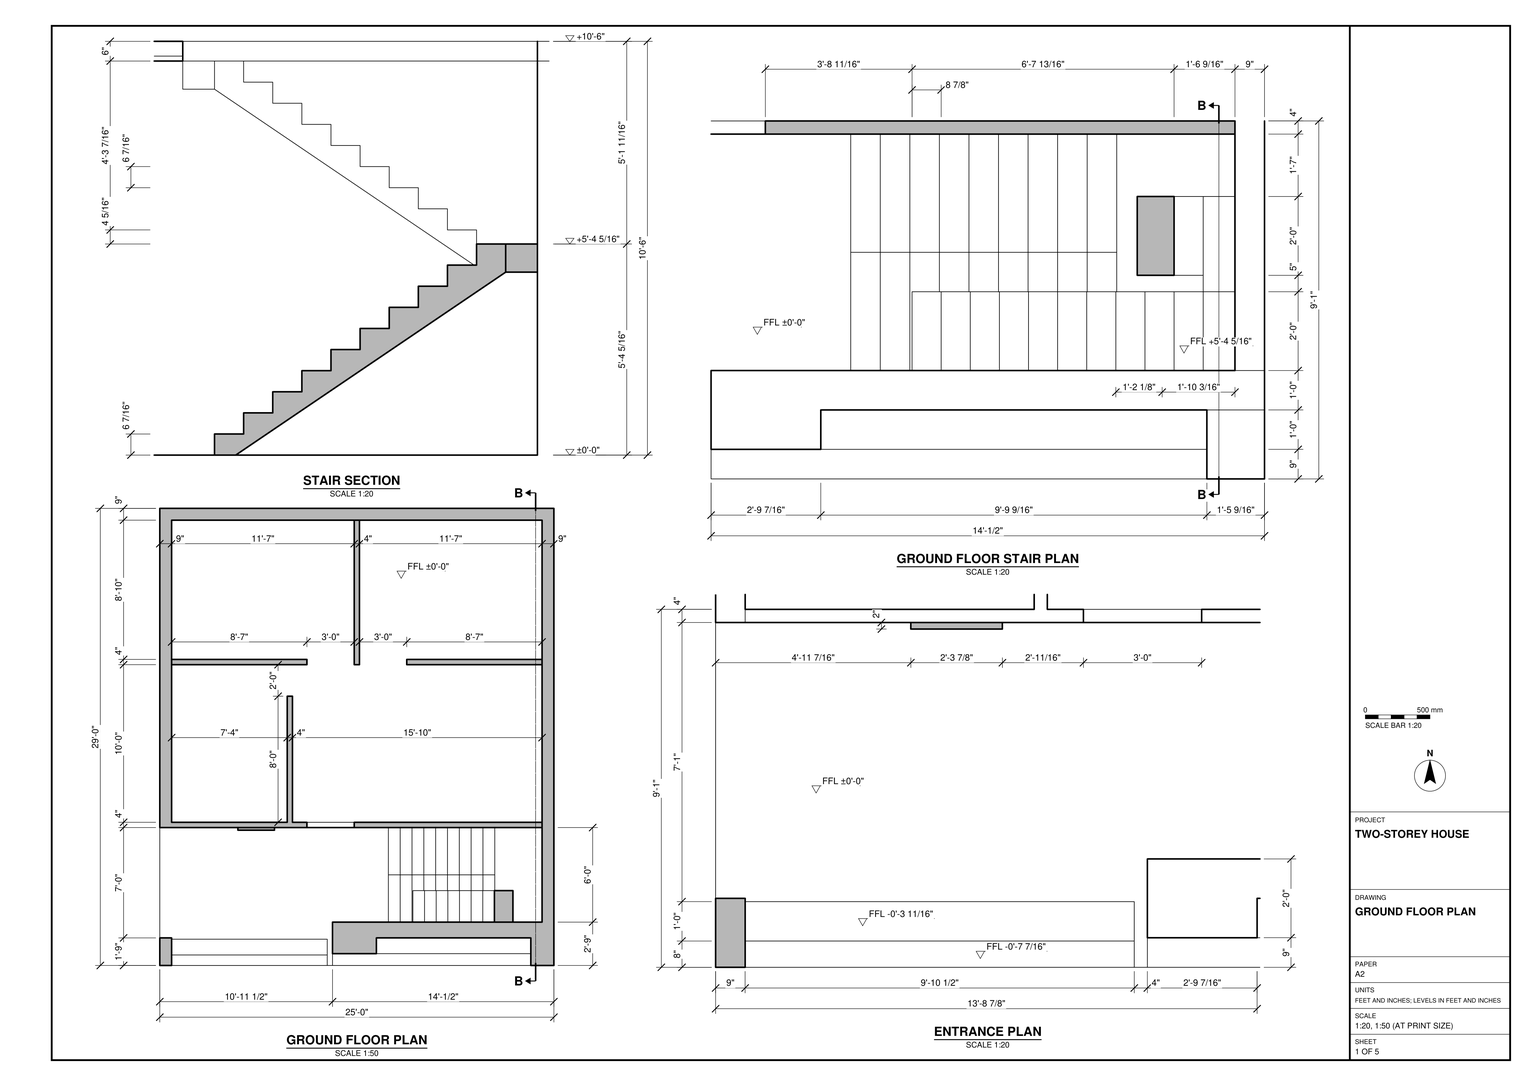
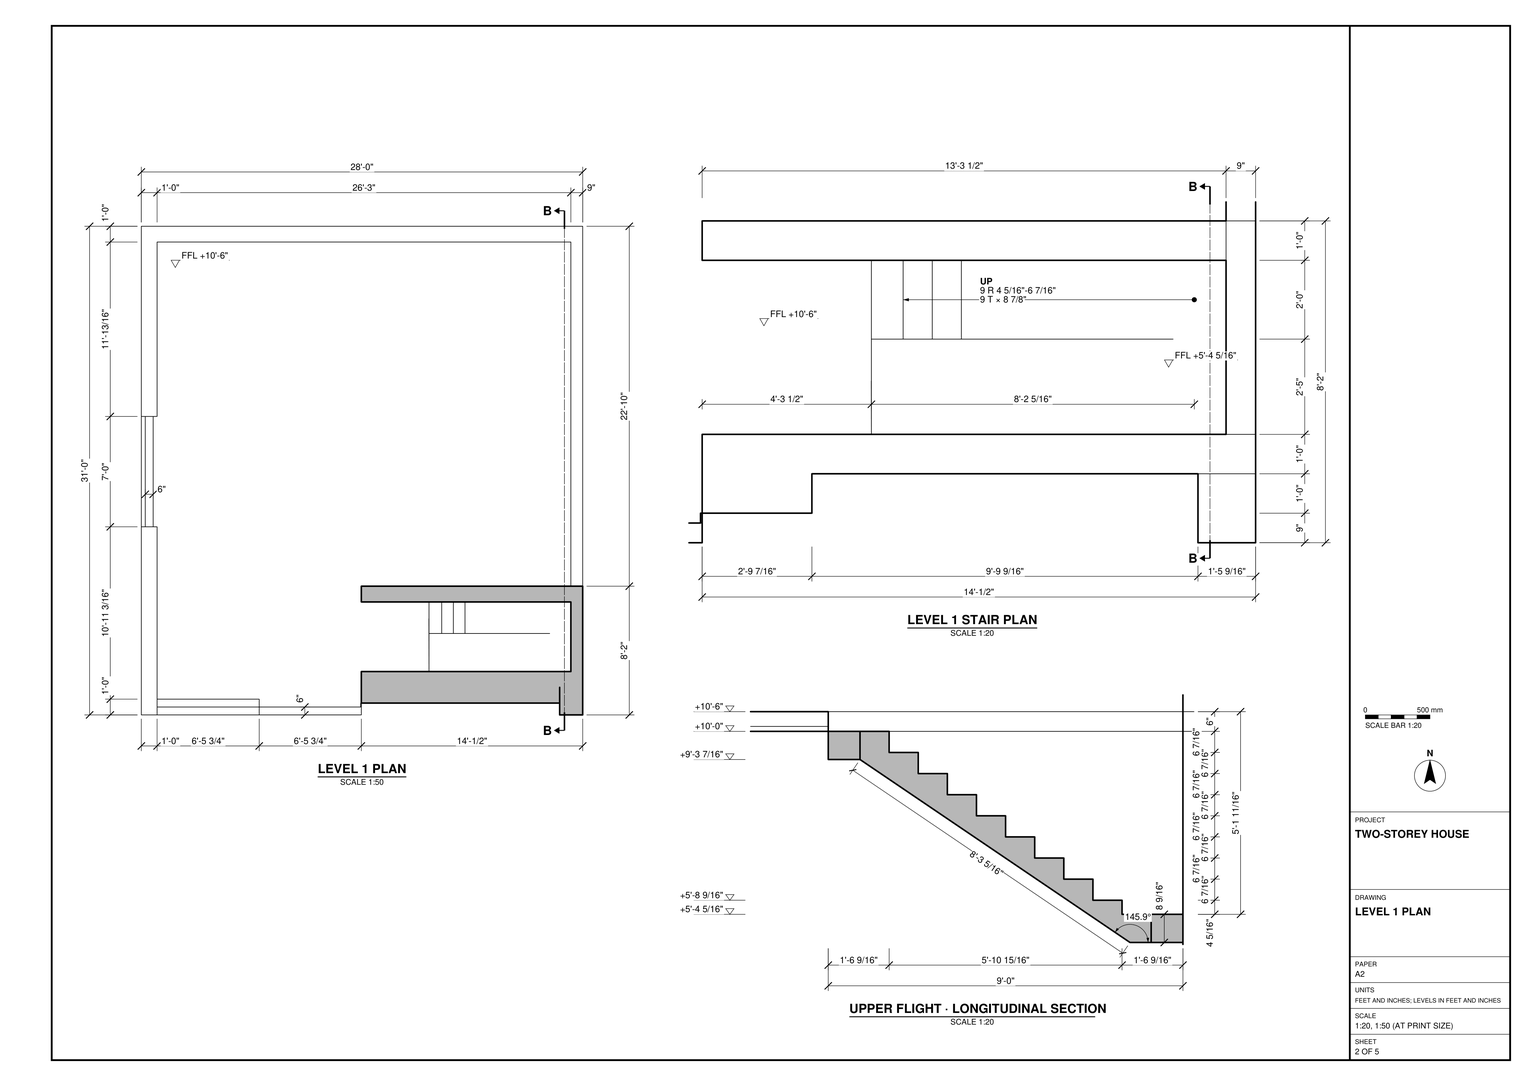
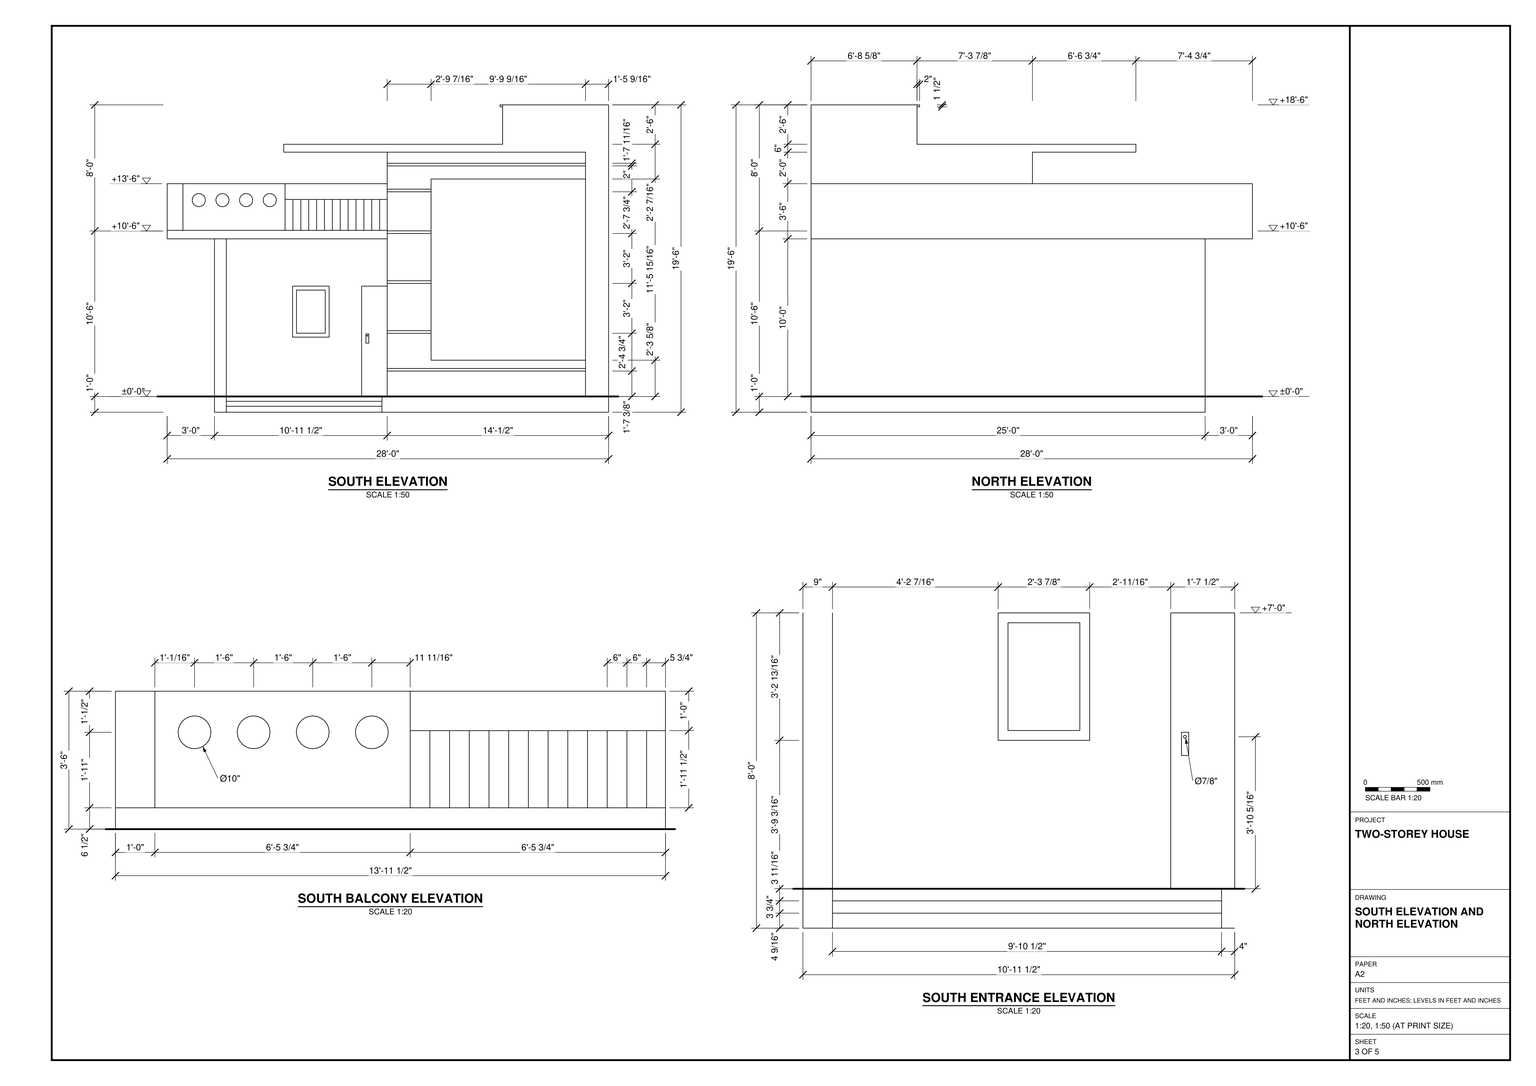
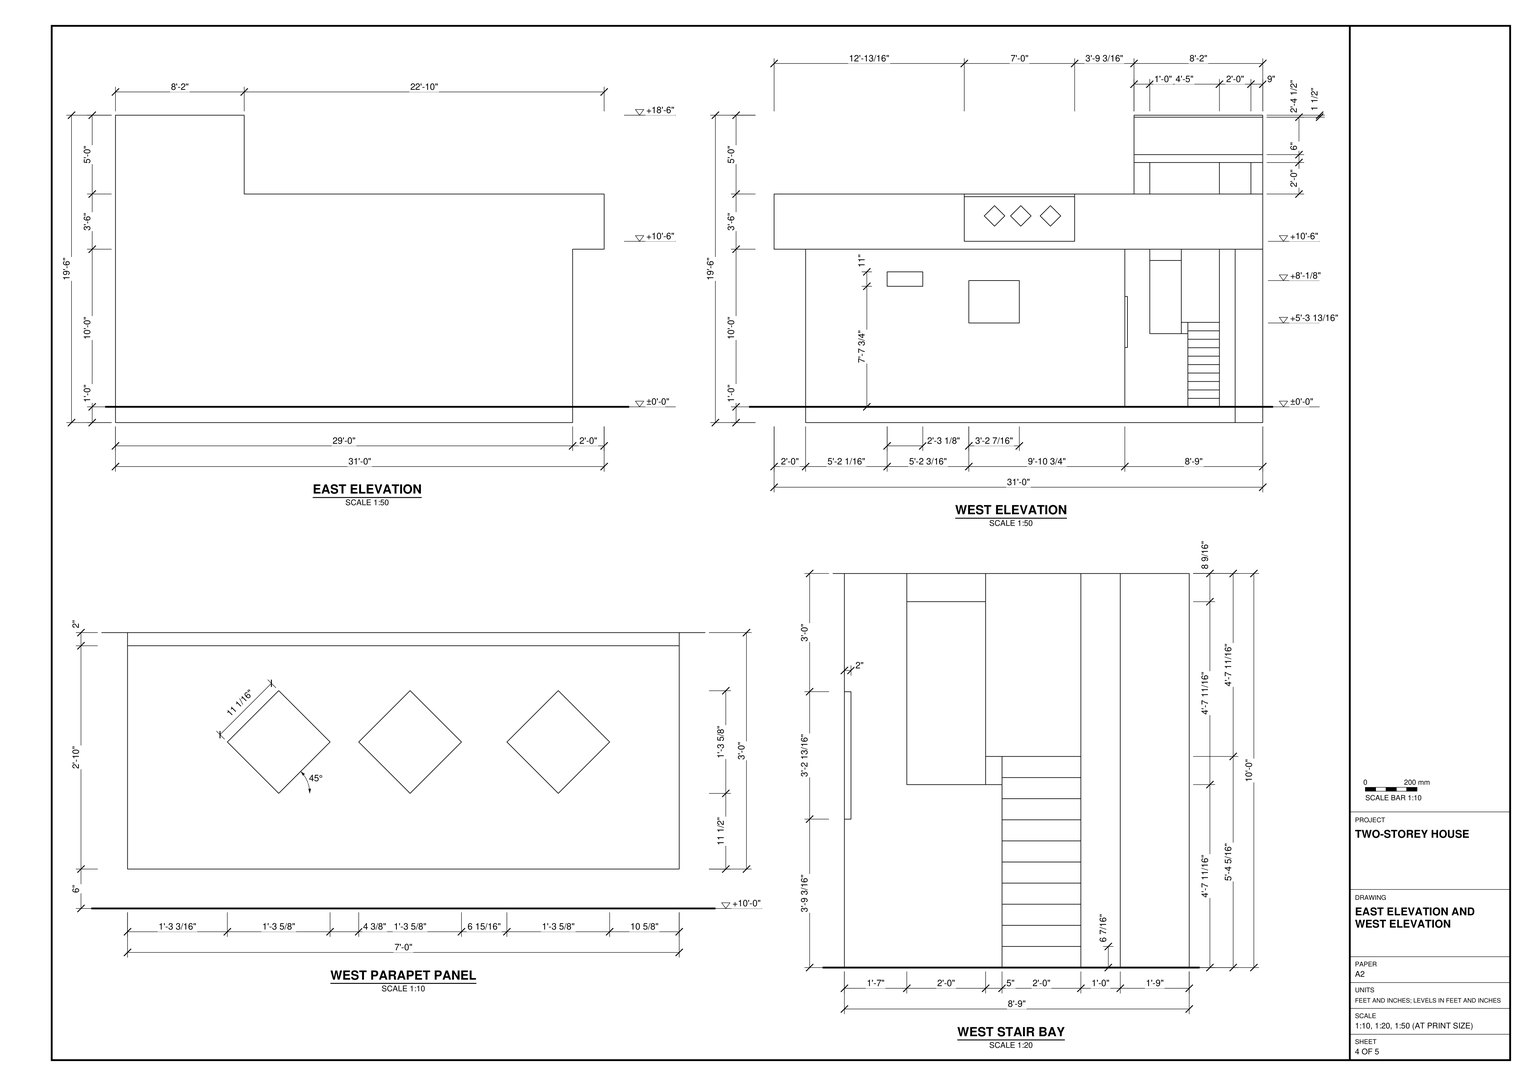
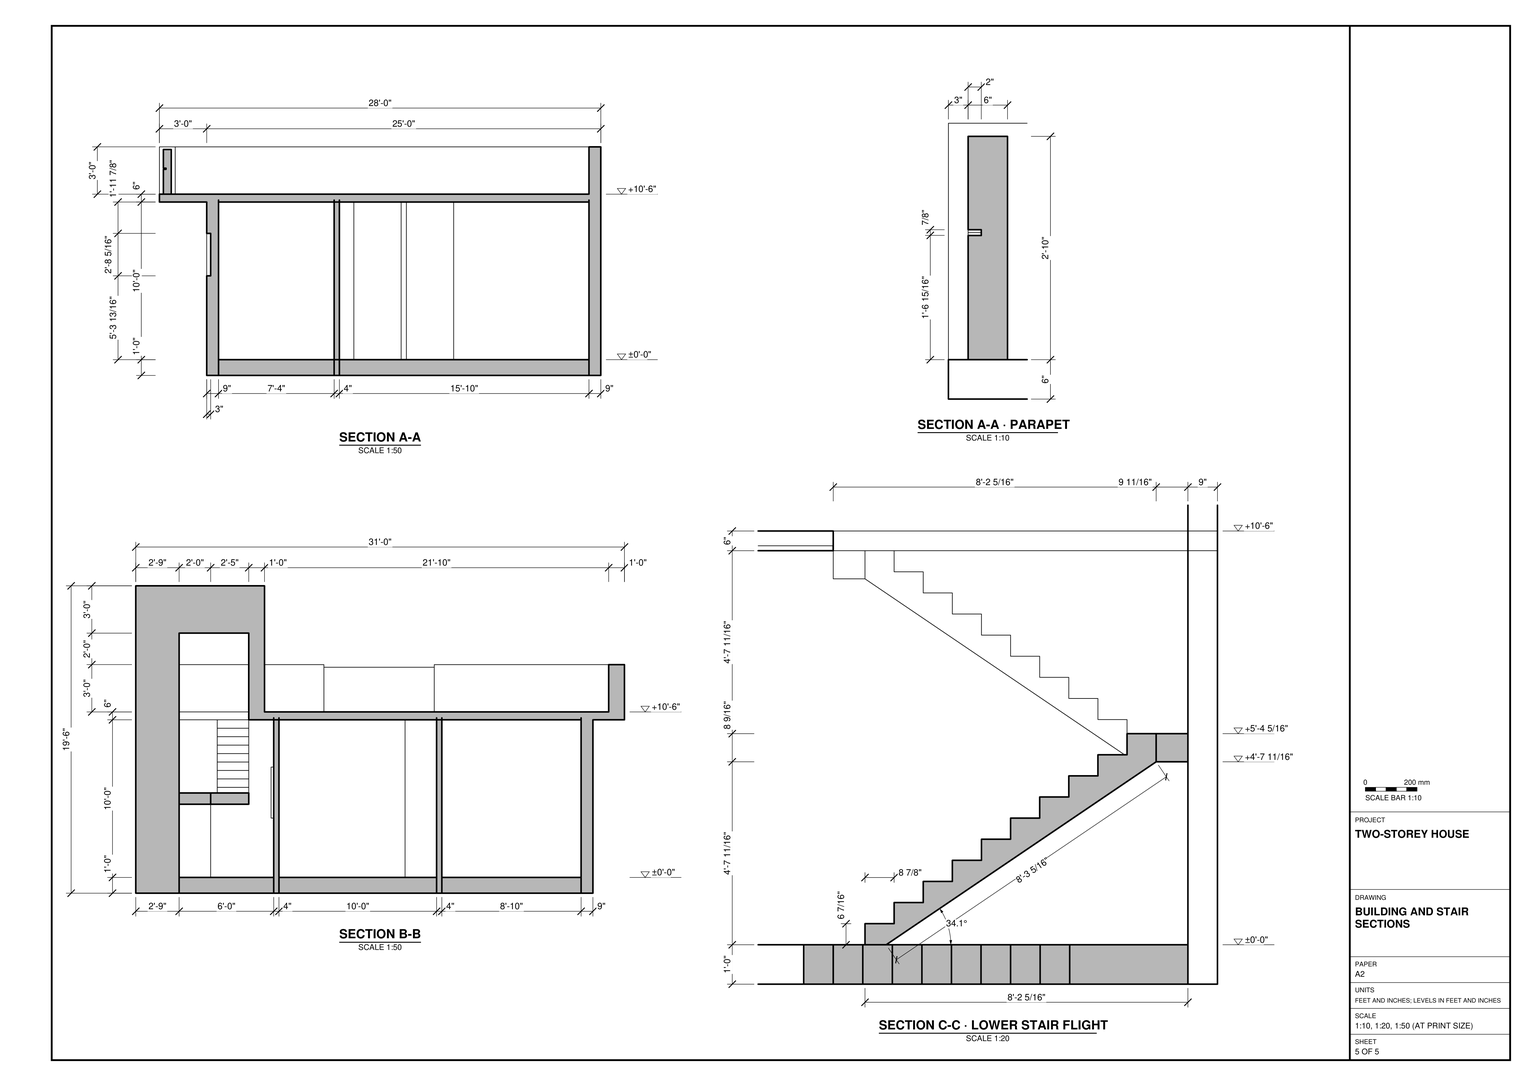
Build the house in SketchUp from task_files/diagram_01.pdf. Work in feet and inches. The complete model extents are 63'-3 1/16" along X, 31'-11 3/16" along Y and 19'-6" vertically. Use the plan dimensions for the house itself: the ground-floor footprint, including the entrance and stair area, is 25'-0" by 29'-0". Set the ground floor at ±0'-0" and the upper level at +10'-6".

Model the base, floor slabs, 9" exterior walls and 4" interior partitions. Follow the ground-floor plan for the paired rear rooms, the shorter partition in front of them and the gaps that give access between spaces. Recess the south entrance behind the balcony, with steps up to the door and a framed window to its left. Beside the entrance, build the two stair flights running in opposite directions, joined at the +5'-4 5/16" landing. Match the stepped treads and inclined undersides in section, and leave the opening for arrival at the roof terrace.

Follow the elevations for the projecting upper slab, terrace edges and taller stepped surround beside the stair. On the south balcony, distinguish the panel with circular details from the adjoining vertical railing. Keep walls, slabs, roof elements and stairs in separate groups or components; keep each furniture or joinery piece shown separate and use components for repeated parts. Any decor or loose items shown may be suitable library components. Save one SketchUp model as output_files/two_storey_house_with_its_return_stair_and_roof_terrace.skp.

# SketchUp Ruby script. Lengths in inches.
U = 1.inch
M = Sketchup.active_model
def pt(a) = Geom::Point3d.new(a.map { |v| v * U })
def face(e, loops, mat)
  f = e.add_face(loops[0].map { |a| pt(a) })
  loops[1..].each { |l| e.add_face(l.map { |a| pt(a) }).erase! }
  f.material = f.back_material = mat if mat
  f
end
# faces: each face lists its corners as indices into pts; further lists are holes
def faces(e, pts, list, mat = nil) = list.each { |f| face(e, (f[0].is_a?(Array) ? f : [f]).map { |l| l.map { |i| pts[i] } }, mat) }
# xy, xz, yz: faces in a plane at the given z, y or x. An outline is a flat list of corners, or four numbers for a rectangle; further outlines are holes
def ring(l) = l.size == 4 ? [[l[0], l[1]], [l[2], l[1]], [l[2], l[3]], [l[0], l[3]]] : l.each_slice(2).to_a
def flat(e, list, mat, &to3) = list.each { |f| face(e, (f[0].is_a?(Array) ? f : [f]).map { |l| ring(l).map { |u, v| to3.(u, v) } }, mat) }
def xy(e, z, list, mat = nil) = flat(e, list, mat) { |x, y| [x, y, z] }
def xz(e, y, list, mat = nil) = flat(e, list, mat) { |x, z| [x, y, z] }
def yz(e, x, list, mat = nil) = flat(e, list, mat) { |y, z| [x, y, z] }
def lines(e, pts, list) = list.each { |a, b| e.add_line(pt(pts[a]), pt(pts[b])) }
# prism: a flat outline (further loops are holes) pulled along v
def prism(e, loops, v, mat = nil)
  f = face(e, loops, mat); d = Geom::Vector3d.new(v.map { |x| x * U })
  f.pushpull(f.normal.samedirection?(d) ? d.length : -d.length)
end
def box(e, o, s, mat = nil) = prism(e, [[o, [o[0] + s[0], o[1], o[2]], [o[0] + s[0], o[1] + s[1], o[2]], [o[0], o[1] + s[1], o[2]]]], [0, 0, s[2]], mat)
def at(x, y, z, deg = 0) = Geom::Transformation.translation(pt([x, y, z])) * Geom::Transformation.rotation(ORIGIN, Z_AXIS, deg.degrees)
def axes(o, x, y, z) = Geom::Transformation.new([*x, 0, *y, 0, *z, 0, *pt(o).to_a, 1])
def part(name) = M.definitions.add(name)
# library, detail: a bought-in or finely detailed component or shape, given as its bounding box
def library(name, o, s) = part(name).tap { |d| box(d.entities, o, s) }
def detail(e, o, s) = box(e.add_group.entities, o, s)
def put(e, d, t, mat = nil) = e.add_instance(d, t).tap { |i| i.material = mat if mat }
def group(e, t, mat = nil) = e.add_group.tap { |g| g.transformation = t; g.material = mat if mat }.entities
root = M.entities
M.materials.add("[0006_Pink]").color = [255, 192, 203]
M.materials.add("[0017_IndianRed]").color = [205, 92, 92]
M.materials.add("[0022_Maroon]").color = [58, 0, 0]
M.materials.add("[0078_DarkSlateGray]").color = [47, 79, 79]
M.materials.add("[0081_CadetBlue]").color = [43, 73, 73]
M.materials.add("[0081_CadetBlue]1").color = [78, 130, 132]
M.materials.add("[0081_CadetBlue]2").color = [69, 115, 117]
M.materials.add("[0093_AliceBlue]").color = [240, 248, 255]
M.materials.add("[0099_LightSteelBlue]").color = [176, 196, 222]
M.materials.add("[0117_GhostWhite]").color = [248, 248, 255]
M.materials.add("[0118_Thistle]").color = [198, 175, 198]
M.materials.add("[0119_RosyBrown]").color = [247, 188, 188]
M.materials.add("[Grass Dark Green]").color = [106, 157, 55]
M.materials.add("[Stone Marble]").color = [143, 138, 136]
M.materials.add("[Stone Vein Gray]").color = [166, 165, 165]
M.materials.add("[Translucent Resin Crush Gray]").color = [184, 184, 184]
M.materials["[Translucent Resin Crush Gray]"].alpha = 0.8
M.materials.add("[Wood Veneer 01]").color = [84, 49, 25]
M.materials.add("[Wood Veneer 01]1").color = [120, 70, 37]
xy(root,-12,[[36,0,45,21],[45,0,163.47,9],[163.47,0,167.47,33],[167.47,0,336,33],[45,9,163.47,21],
  [36,21,163.47,33],[327,33,327,339,45,339,45,105,36,105,36,348,336,348,336,33],[36,33,36,105,148,105,148,109,137,109,137,205,133,205,133,109,45,109,45,229,148,229,148,233,45,233,45,339,184,339,184,229,188,229,188,339,327,339,327,233,224,233,224,229,327,229,327,109,184,109,184,105,210,105,210,33],[210,33,219,69],[219,33,228,69],
  [228,33,237,69],[237,33,246,69],[246,33,255,69],[255,33,264,69],[264,33,273,69],
  [273,33,282,69],[282,33,291,69],[291,33,327,105],[210,69,219,105],[219,69,228,105],
  [228,69,237,105],[237,69,246,105],[246,69,255,105],[255,69,264,105],[264,69,273,105],
  [273,69,282,105],[282,69,291,105],[45,105,45,109,133,109,133,205,137,205,137,109,148,109,148,105],[184,105,327,109],[45,229,148,233],
  [184,229,188,339],[224,229,327,233]])
xy(root,-7.4375,[[45,8,163.47,9]])
xy(root,-7.4375,[[45,0,163.47,8]],"[Stone Marble]")
xy(root,-3.6875,[[45,20,163.47,21]])
xy(root,-3.6875,[[45,8,163.47,20]],"[Stone Marble]")
xy(root,0,[[210,33,219,69],[219,33,228,69],[228,33,237,69],[237,33,246,69],[246,33,255,69],
  [255,33,264,69],[264,33,273,69],[273,33,282,69],[282,33,291,69],[291,33,327,105],
  [459.09,35.21,468.09,195.77],[468.09,35.21,586.56,44.21],[586.56,35.21,590.56,68.21],[590.56,35.21,759.09,68.21],[468.09,44.21,586.56,56.21],
  [468.09,56.21,586.56,68.21],[750.09,68.21,759.09,68.21,759.09,383.21,459.09,383.21,459.09,219.77,468.09,219.77,468.09,374.21,750.09,374.21],[468.09,68.21,633.09,68.21,633.09,140.21,607.09,140.21,607.09,144.21,750.09,144.21,750.09,264.21,647.09,264.21,647.09,268.21,750.09,268.21,750.09,374.21,611.09,374.21,611.09,264.21,607.09,264.21,607.09,374.21,468.09,374.21,468.09,268.21,571.09,268.21,571.09,264.21,468.09,264.21,468.09,144.21,556.09,144.21,556.09,240.21,560.09,240.21,560.09,144.21,571.09,144.21,571.09,140.21,468.09,140.21],[633.09,68.21,642.09,104.21],[642.09,68.21,651.09,104.21],
  [651.09,68.21,660.09,104.21],[660.09,68.21,669.09,104.21],[669.09,68.21,678.09,104.21],[678.09,68.21,687.09,104.21],[687.09,68.21,696.09,104.21],
  [696.09,68.21,705.09,104.21],[705.09,68.21,714.09,104.21],[714.09,68.21,750.09,140.21],[210,69,219,105],[219,69,228,105],
  [228,69,237,105],[237,69,246,105],[246,69,255,105],[255,69,264,105],[264,69,273,105],
  [273,69,282,105],[282,69,291,105],[633.09,104.21,642.09,140.21],[642.09,104.21,651.09,140.21],[651.09,104.21,660.09,140.21],
  [660.09,104.21,669.09,140.21],[669.09,104.21,678.09,140.21],[678.09,104.21,687.09,140.21],[687.09,104.21,696.09,140.21],[696.09,104.21,705.09,140.21],
  [705.09,104.21,714.09,140.21],[45,105,148,105,148,109,137,109,137,205,133,205,133,109,45,109],[148,105,184,109],[45,109,133,109,133,205,137,205,137,109,327,109,327,229,224,229,224,233,327,233,327,339,188,339,188,229,184,229,184,339,45,339,45,233,148,233,148,229,45,229],[468.09,140.21,495.28,144.21],
  [495.28,140.21,519.28,142.21],[519.28,140.21,571.09,140.21,571.09,144.21,560.09,144.21,560.09,240.21,556.09,240.21,556.09,144.21,519.28,144.21],[607.09,140.21,750.09,144.21],[495.28,142.21,519.28,144.21],[459.09,195.77,463.59,219.77],
  [463.59,195.77,468.09,219.77],[184,229,188,339],[468.09,264.21,571.09,268.21],[607.09,264.21,611.09,374.21],[647.09,264.21,750.09,268.21]])
xy(root,0,[[167.47,0,318.45,9]],"[Grass Dark Green]")
xy(root,0,[[163.47,0,167.47,0,167.47,33,210,33,210,105,36,105,36,21,45,21,45,20,163.47,20]],"[Stone Vein Gray]")
xy(root,27.62,[[200.89,9,318.45,21]],"[0081_CadetBlue]")
xy(root,45.1875,[[95.4375,103,123.3125,105]],"[Wood Veneer 01]1")
xy(root,48.1875,[[98.4375,103,120.3125,105]],"[Wood Veneer 01]1")
xy(root,63.8125,[[36,185.32,39,223.76]])
xy(root,81,[[98.4375,103,120.3125,105]],"[Wood Veneer 01]1")
xy(root,84,[[148,105,184,109]])
xy(root,84,[[95.4375,103,123.3125,105]],"[Wood Veneer 01]1")
xy(root,91.76,[[36,258.82,38,285.95]])
xy(root,96.125,[[36,185.32,39,223.76]])
xy(root,102.76,[[36,258.82,38,285.95]])
xy(root,120,[[219,33,218.87,86,219,86],[77.91,34.22,76.38,34.55,74.99,35.28,73.83,36.34,72.99,37.66,72.52,39.15,72.45,40.72,72.79,42.25,73.52,43.63,74.57,44.79,75.9,45.63,77.39,46.1,78.95,46.17,80.48,45.83,81.87,45.11,83.03,44.05,83.87,42.73,84.34,41.23,84.41,39.67,84.07,38.14,83.35,36.75,82.29,35.6,80.97,34.75,79.47,34.28],[124.78,34.22,123.25,34.55,121.86,35.28,120.71,36.34,119.87,37.66,119.4,39.15,119.33,40.72,119.67,42.25,120.39,43.63,121.45,44.79,122.77,45.63,124.26,46.1,125.83,46.17,127.36,45.83,128.75,45.11,129.9,44.05,130.74,42.73,131.21,41.23,131.28,39.67,130.94,38.14,130.22,36.75,129.16,35.6,127.84,34.75,126.35,34.28],[45,105,45,109,133,109,133,205,137,205,137,109,148,109,148,105],[148,105,184,109],
  [184,105,327,109],[45,109,45,229,148,229,148,233,45,233,45,339,184,339,184,229,188,229,188,339,327,339,327,233,224,233,224,229,327,229,327,109,137,109,137,205,133,205,133,109],[45,229,148,233],[184,229,188,339],[224,229,327,233],
  [36,348,336,372]])
xy(root,120,[[[0,0,0,372,36,372,36,105,327,105,327,86,218.87,86,219,33,167.47,33,167.47,0,45,0,45,21,36,21,36,0],[124.78,34.22,126.35,34.28,127.84,34.75,129.16,35.6,130.22,36.75,130.94,38.14,131.28,39.67,131.21,41.23,130.74,42.73,129.9,44.05,128.75,45.11,127.36,45.83,125.83,46.17,124.26,46.1,122.77,45.63,121.45,44.79,120.39,43.63,119.67,42.25,119.33,40.72,119.4,39.15,119.87,37.66,120.71,36.34,121.86,35.28,123.25,34.55],[77.91,34.22,79.47,34.28,80.97,34.75,82.29,35.6,83.35,36.75,84.07,38.14,84.41,39.67,84.34,41.23,83.87,42.73,83.03,44.05,81.87,45.11,80.48,45.83,78.95,46.17,77.39,46.1,75.9,45.63,74.57,44.79,73.52,43.63,72.79,42.25,72.45,40.72,72.52,39.15,72.99,37.66,73.83,36.34,74.99,35.28,76.38,34.55]]],"[0118_Thistle]")
xy(root,126,[[89.74,6,166.97,6,166.97,9,167.47,9,167.47,33,219,33,219,86,167.47,86,167.47,98,327,98,327,360,12,360,12,227.21,9,227.21,9,143.21,12,143.21,12,12,89.74,12],[166.97,6,167.47,9],[3,143.21,9,227.21]])
xy(root,126,[[0,143.21,3,227.21]],"[0081_CadetBlue]2")
xy(root,126.5,[[95.74,0,101.74,2],[107.74,0,113.74,2],[119.74,0,125.74,2],[131.74,0,137.74,2],[143.74,0,149.74,2],
  [155.74,0,161.74,2]])
xy(root,126.5,[[12,0,89.74,6]],"[0078_DarkSlateGray]")
xy(root,150,[[89.74,0,95.74,0,95.74,2,101.74,2,101.74,6,89.74,6],[95.74,0,101.74,2],[101.74,0,107.74,6],[107.74,0,113.74,2],[113.74,0,119.74,6],
  [119.74,0,125.74,2],[125.74,0,131.74,6],[131.74,0,137.74,2],[137.74,0,143.74,6],[143.74,0,149.74,2],
  [149.74,0,155.74,6],[155.74,0,161.74,2],[107.74,2,113.74,6],[119.74,2,125.74,6],[131.74,2,137.74,6],
  [143.74,2,149.74,6],[155.74,2,161.74,6]])
xy(root,160,[[3,143.21,9,227.21]],"[Wood Veneer 01]1")
xy(root,162,[[0,0,12,143.21],[12,6,89.74,12],[166.97,6,167.47,9],[327,98,336,98,336,372,0,372,0,227.21,12,227.21,12,360,327,360]])
xy(root,162,[[89.74,0,167.47,6]],"[0017_IndianRed]")
xy(root,165.56,[[200.89,9,318.45,21]],"[0081_CadetBlue]")
xy(root,186,[[167.47,9,318.45,21]])
xy(root,186,[[[88.72,0,88.72,98,167.47,98,167.47,86,327,86,327,33,167.47,33,167.47,9,318.45,9,318.45,0],[122.65,43.52,124.89,43.55,127.11,43.82,129.29,44.32,131.41,45.04,133.43,45.98,135.36,47.13,137.14,48.47,138.78,50,140.26,51.68,141.54,53.51,142.63,55.47,143.51,57.52,144.17,59.66,144.6,61.86,144.8,64.08,144.77,66.32,144.5,68.54,144,70.72,143.28,72.84,142.33,74.87,141.1875,76.79,139.84,78.58,138.32,80.22,136.64,81.69,134.81,82.98,132.85,84.07,130.79,84.95,128.66,85.61,126.46,86.04,124.23,86.24,121.99,86.2,119.77,85.93,117.59,85.44,115.47,84.71,113.45,83.77,111.52,82.62,109.74,81.28,108.1,79.76,106.625,78.07,105.34,76.24,104.25,74.29,103.37,72.23,102.71,70.09,102.28,67.9,102.08,65.67,102.11,63.43,102.38,61.21,102.88,59.03,103.6,56.91,104.55,54.88,105.69,52.96,107.04,51.17,108.56,49.53,110.24,48.06,112.07,46.77,114.03,45.68,116.09,44.81,118.22,44.15,120.42,43.72]]],"[Wood Veneer 01]1")
xy(root,192,[[[88.72,0,255.36,98],[122.65,43.52,120.42,43.72,118.22,44.15,116.09,44.81,114.03,45.68,112.07,46.77,110.24,48.06,108.56,49.53,107.04,51.17,105.69,52.96,104.55,54.88,103.6,56.91,102.88,59.03,102.38,61.21,102.11,63.43,102.08,65.67,102.28,67.9,102.71,70.09,103.37,72.23,104.25,74.29,105.34,76.24,106.625,78.07,108.1,79.76,109.74,81.28,111.52,82.62,113.45,83.77,115.47,84.71,117.59,85.44,119.77,85.93,121.99,86.2,124.23,86.24,126.46,86.04,128.66,85.61,130.79,84.95,132.85,84.07,134.81,82.98,136.64,81.69,138.32,80.22,139.84,78.58,141.1875,76.79,142.33,74.87,143.28,72.84,144,70.72,144.5,68.54,144.77,66.32,144.8,64.08,144.6,61.86,144.17,59.66,143.51,57.52,142.63,55.47,141.54,53.51,140.26,51.68,138.78,50,137.14,48.47,135.36,47.13,133.43,45.98,131.41,45.04,129.29,44.32,127.11,43.82,124.89,43.55]]],"[0006_Pink]")
xy(root,220.5,[[253.36,0,255.36,98]],"[0006_Pink]")
xy(root,222,[[253.36,0,336,98]],"[0006_Pink]")
xz(root,0,[[0,120,167.47,126.5],[89.74,126.5,95.74,150],[101.74,126.5,107.74,150],[113.74,126.5,119.74,150],[125.74,126.5,131.74,150],
  [137.74,126.5,143.74,150],[149.74,126.5,155.74,150],[161.74,126.5,167.47,150]])
xz(root,0,[[253.36,220.5,255.36,222]],"[0006_Pink]")
xz(root,0,[[89.74,150,167.47,162]],"[0017_IndianRed]")
xz(root,0,[[0,126.5,12,162]],"[0078_DarkSlateGray]")
xz(root,0,[[36,-12,45,120]],"[0081_CadetBlue]1")
xz(root,0,[[163.47,-12,336,-12,336,222,255.36,222,255.36,192,88.72,192,88.72,186,318.45,186,318.45,0,163.47,0]],"[0119_RosyBrown]")
xz(root,0,[[45,-12,163.47,-7.4375]],"[Stone Marble]")
xz(root,2,[[95.74,126.5,101.74,150],[107.74,126.5,113.74,150],[119.74,126.5,125.74,150],[131.74,126.5,137.74,150],[143.74,126.5,149.74,150],
  [155.74,126.5,161.74,150]])
xz(root,6,[[12,126,89.74,126.5],[89.74,126,166.97,150],[24.07,144.5,25.37,144.67,26.57,145.17,27.61,145.96,28.4,147,28.9,148.2,29.07,149.5,28.9,150.79,28.4,152,27.61,153.03,26.57,153.83,25.37,154.33,24.07,154.5,22.78,154.33,21.57,153.83,20.54,153.03,19.74,152,19.24,150.79,19.07,149.5,19.24,148.2,19.74,147,20.54,145.96,21.57,145.17,22.78,144.67],[42.07,144.5,43.37,144.67,44.57,145.17,45.61,145.96,46.4,147,46.9,148.2,47.07,149.5,46.9,150.79,46.4,152,45.61,153.03,44.57,153.83,43.37,154.33,42.07,154.5,40.78,154.33,39.57,153.83,38.54,153.03,37.74,152,37.24,150.79,37.07,149.5,37.24,148.2,37.74,147,38.54,145.96,39.57,145.17,40.78,144.67],[60.07,144.5,61.37,144.67,62.57,145.17,63.61,145.96,64.4,147,64.9,148.2,65.07,149.5,64.9,150.79,64.4,152,63.61,153.03,62.57,153.83,61.37,154.33,60.07,154.5,58.78,154.33,57.57,153.83,56.54,153.03,55.74,152,55.24,150.79,55.07,149.5,55.24,148.2,55.74,147,56.54,145.96,57.57,145.17,58.78,144.67],
  [78.07,144.5,79.37,144.67,80.57,145.17,81.61,145.96,82.4,147,82.9,148.2,83.07,149.5,82.9,150.79,82.4,152,81.61,153.03,80.57,153.83,79.37,154.33,78.07,154.5,76.78,154.33,75.57,153.83,74.54,153.03,73.74,152,73.24,150.79,73.07,149.5,73.24,148.2,73.74,147,74.54,145.96,75.57,145.17,76.78,144.67],[89.74,150,166.97,162]])
xz(root,6,[[[12,126.5,89.74,162],[78.07,144.5,76.78,144.67,75.57,145.17,74.54,145.96,73.74,147,73.24,148.2,73.07,149.5,73.24,150.79,73.74,152,74.54,153.03,75.57,153.83,76.78,154.33,78.07,154.5,79.37,154.33,80.57,153.83,81.61,153.03,82.4,152,82.9,150.79,83.07,149.5,82.9,148.2,82.4,147,81.61,145.96,80.57,145.17,79.37,144.67],[60.07,144.5,58.78,144.67,57.57,145.17,56.54,145.96,55.74,147,55.24,148.2,55.07,149.5,55.24,150.79,55.74,152,56.54,153.03,57.57,153.83,58.78,154.33,60.07,154.5,61.37,154.33,62.57,153.83,63.61,153.03,64.4,152,64.9,150.79,65.07,149.5,64.9,148.2,64.4,147,63.61,145.96,62.57,145.17,61.37,144.67],[24.07,144.5,22.78,144.67,21.57,145.17,20.54,145.96,19.74,147,19.24,148.2,19.07,149.5,19.24,150.79,19.74,152,20.54,153.03,21.57,153.83,22.78,154.33,24.07,154.5,25.37,154.33,26.57,153.83,27.61,153.03,28.4,152,28.9,150.79,29.07,149.5,28.9,148.2,28.4,147,27.61,145.96,26.57,145.17,25.37,144.67],[42.07,144.5,40.78,144.67,39.57,145.17,38.54,145.96,37.74,147,37.24,148.2,37.07,149.5,37.24,150.79,37.74,152,38.54,153.03,39.57,153.83,40.78,154.33,42.07,154.5,43.37,154.33,44.57,153.83,45.61,153.03,46.4,152,46.9,150.79,47.07,149.5,46.9,148.2,46.4,147,45.61,145.96,44.57,145.17,43.37,144.67]]],"[0078_DarkSlateGray]")
xz(root,8,[[45,-7.4375,163.47,-3.6875]],"[Stone Marble]")
xz(root,9,[[45,-12,163.47,-7.4375],[167.47,19.34,318.45,21.34],[167.47,48.09,200.89,50.09],[167.47,86.09,200.89,88.09],[167.47,124.09,200.89,126.09],
  [166.97,126,167.47,162],[167.47,155.83,200.89,157.83],[167.47,175.53,318.45,177.53]])
xz(root,9,[[167.47,0,318.45,19.34],[167.47,21.34,318.45,21.34,318.45,27.62,200.89,27.62,200.89,48.09,167.47,48.09],[167.47,50.09,200.89,86.09],[167.47,88.09,200.89,124.09],[167.47,126.09,200.89,155.83],
  [167.47,157.83,200.89,157.83,200.89,165.56,318.45,165.56,318.45,175.53,167.47,175.53],[167.47,177.53,318.45,186]],"[0081_CadetBlue]")
xz(root,12,[[12,126,89.74,162]])
xz(root,20,[[45,-3.6875,163.47,0]],"[Stone Marble]")
xz(root,21,[[36,-12,45,0],[45,-12,163.47,-3.6875]])
xz(root,21,[[36,0,45,120]],"[0081_CadetBlue]1")
xz(root,21,[[200.89,27.62,318.45,165.56]],"[Wood Veneer 01]")
xz(root,33,[[167.47,-12,210,0],[210,-12,219,0],[219,-12,228,0],[228,-12,237,0],[237,-12,246,0],
  [246,-12,255,0],[255,-12,264,0],[264,-12,273,0],[273,-12,282,0],[282,-12,291,0],
  [291,-12,327,0],[167.47,126,327,186]])
xz(root,33,[[167.47,0,167.47,120,219,120,219,126,327,126,327,0]],"[0081_CadetBlue]1")
xz(root,69,[[210,-12,219,0],[219,-12,228,0],[228,-12,237,0],[237,-12,246,0],[246,-12,255,0],
  [255,-12,264,0],[264,-12,273,0],[273,-12,282,0],[282,-12,291,0]])
xz(root,86,[[218.87,120,218.9,121.5,218.87,121.5],[218.87,120,219,120,219,121.5,218.9,121.5],[219,120,327,126],[218.9,121.5,219,121.5,219,126],[167.47,126,327,186]])
xz(root,98,[[253.36,220.5,255.36,222]])
xz(root,98,[[167.47,126,167.47,186,88.72,186,88.72,192,255.36,192,255.36,222,336,222,336,162,327,162,327,126]],"[0006_Pink]")
xz(root,103,[[[95.4375,45.1875,123.3125,84],[98.4375,48.1875,120.3125,81]]],"[Wood Veneer 01]1")
xz(root,105,[[45,-12,148,0],[184,-12,210,0],[210,-12,219,0],[219,-12,228,0],[228,-12,237,0],
  [237,-12,246,0],[246,-12,255,0],[255,-12,264,0],[264,-12,273,0],[273,-12,282,0],
  [282,-12,291,0],[291,-12,327,0],[[95.4375,45.1875,123.3125,84],[98.4375,48.1875,120.3125,81]],[45,120,148,121.5],[184,120,327,121.5]])
xz(root,105,[[[148,0,184,84],[170.08,18.88,176.83,74.32],[151.27,40.59,153.46,47.65]]],"[0022_Maroon]")
xz(root,105,[[170.08,18.88,176.83,74.32],[[151.27,40.59,153.46,47.65],[152.3125,45.85,152.2,45.86,152.1,45.91,152,45.98,151.94,46.07,151.89,46.17,151.875,46.28,151.89,46.4,151.94,46.5,152,46.59,152.1,46.66,152.2,46.71,152.3125,46.72,152.43,46.71,152.53,46.66,152.625,46.59,152.69,46.5,152.74,46.4,152.75,46.28,152.74,46.17,152.69,46.07,152.625,45.98,152.53,45.91,152.43,45.86]],[152.3125,45.85,152.43,45.86,152.53,45.91,152.625,45.98,152.69,46.07,152.74,46.17,152.75,46.28,152.74,46.4,152.69,46.5,152.625,46.59,152.53,46.66,152.43,46.71,152.3125,46.72,152.2,46.71,152.1,46.66,152,46.59,151.94,46.5,151.89,46.4,151.875,46.28,151.89,46.17,151.94,46.07,152,45.98,152.1,45.91,152.2,45.86]],"[0093_AliceBlue]")
xz(root,105,[[[36,0,148,0,148,84,184,84,184,0,327,0,327,120,36,120],[95.4375,45.1875,123.3125,84]]],"[0099_LightSteelBlue]")
xz(root,105,[[98.4375,48.1875,120.3125,81]],"[Translucent Resin Crush Gray]")
xz(root,109,[[45,-12,133,0],[137,-12,148,0],[184,-12,327,0],[45,0,133,120],[137,0,148,120],
  [148,0,184,2],[184,0,327,120],[148,84,184,120],[45,120,133,121.5],[137,120,148,121.5],
  [184,120,327,121.5]])
xz(root,143.21,[[0,126,0,162,12,162,12,126,9,126,9,160,3,160,3,126]],"[0081_CadetBlue]2")
xz(root,185.32,[[36,63.8125,39,96.125]])
xz(root,205,[[133,-12,137,0],[133,0,137,120],[133,120,137,121.5]])
xz(root,223.76,[[36,63.8125,39,96.125]])
xz(root,227.21,[[3,126,9,160]])
xz(root,227.21,[[0,126,3,126,3,160,9,160,9,126,12,126,12,162,0,162]],"[0081_CadetBlue]2")
xz(root,229,[[45,-12,148,0],[184,-12,188,0],[224,-12,327,0],[45,0,148,120],[184,0,188,120],
  [224,0,327,120],[45,120,148,121.5],[184,120,188,121.5],[224,120,327,121.5]])
xz(root,233,[[45,-12,148,0],[224,-12,327,0],[45,0,148,120],[224,0,327,120],[45,120,148,121.5],
  [224,120,327,121.5]])
xz(root,258.82,[[36,91.76,38,102.76]])
xz(root,285.95,[[36,91.76,38,102.76]])
xz(root,339,[[45,-12,184,0],[184,-12,188,0],[188,-12,327,0],[45,0,184,120],[184,0,188,120],
  [188,0,327,120],[45,120,184,121.5],[188,120,327,121.5]])
xz(root,348,[[36,-12,336,120]])
xz(root,360,[[12,126,327,162]])
xz(root,372,[[0,120,336,162]])
yz(root,0,[[0,120,0,162,143.21,162,143.21,126,227.21,126,227.21,162,372,162,372,120]],"[0078_DarkSlateGray]")
yz(root,3,[[[143.21,126,227.21,160],[184.19,137.52,192.02,145.35,184.19,153.17,176.37,145.35],[161.63,137.52,169.45,145.35,161.63,153.17,153.81,145.35],[204.19,137.52,212.02,145.35,204.19,153.17,196.37,145.35]]],"[Wood Veneer 01]1")
yz(root,5,[[161.63,137.52,153.81,145.35,161.63,153.17,169.45,145.35],[184.19,137.52,176.37,145.35,184.19,153.17,192.02,145.35],[204.19,137.52,196.37,145.35,204.19,153.17,212.02,145.35]])
yz(root,9,[[143.21,126,227.21,160]],"[Wood Veneer 01]1")
yz(root,12,[[6,126,12,162],[12,126,143.21,162],[227.21,126,360,162]])
yz(root,12,[[0,126.5,6,162]],"[0078_DarkSlateGray]")
yz(root,36,[[[21,-12,21,0,105,0,105,120,348,120,348,-12],[185.32,63.8125,223.76,96.125],[258.82,91.76,285.95,102.76]]])
yz(root,36,[[0,-12,21,120]],"[0081_CadetBlue]1")
yz(root,38,[[258.82,91.76,285.95,102.76]])
yz(root,39,[[185.32,63.8125,223.76,96.125]])
yz(root,45,[[0,-12,9,-7.4375],[9,-12,21,-3.6875],[105,-12,109,0],[109,-12,229,0],[229,-12,233,120],
  [233,-12,339,0],[8,-7.4375,9,-3.6875],[20,-3.6875,21,0],[109,0,229,120],[233,0,339,120],
  [109,120,229,121.5],[233,120,339,121.5]])
yz(root,45,[[0,-7.4375,8,-7.4375,8,-3.6875,20,-3.6875,20,0,21,0,21,120,0,120]],"[0081_CadetBlue]1")
yz(root,88.72,[[0,186,98,192]],"[0119_RosyBrown]")
yz(root,89.74,[[6,126,12,162],[0,126.5,6,150]])
yz(root,89.74,[[0,150,6,162]],"[0017_IndianRed]")
yz(root,95.4375,[[103,45.1875,105,84]],"[Wood Veneer 01]1")
yz(root,95.74,[[0,126.5,2,150]])
yz(root,98.4375,[[103,48.1875,105,81]],"[Wood Veneer 01]1")
yz(root,101.74,[[0,126.5,2,150]])
yz(root,107.74,[[0,126.5,2,150]])
yz(root,113.74,[[0,126.5,2,150]])
yz(root,119.74,[[0,126.5,2,150]])
yz(root,120.3125,[[103,48.1875,105,81]],"[Wood Veneer 01]1")
yz(root,123.3125,[[103,45.1875,105,84]],"[Wood Veneer 01]1")
yz(root,125.74,[[0,126.5,2,150]])
yz(root,131.74,[[0,126.5,2,150]])
yz(root,133,[[109,-12,205,0],[109,0,205,120],[109,120,205,121.5]])
yz(root,137,[[109,-12,205,0],[109,0,205,120],[109,120,205,121.5]])
yz(root,137.74,[[0,126.5,2,150]])
yz(root,143.74,[[0,126.5,2,150]])
yz(root,148,[[105,-12,109,0],[229,-12,233,0],[105,0,109,2],[229,0,233,120],[105,2,109,84],
  [105,120,109,121.5],[229,120,233,121.5]])
yz(root,149.74,[[0,126.5,2,150]])
yz(root,155.74,[[0,126.5,2,150]])
yz(root,161.74,[[0,126.5,2,150]])
yz(root,163.47,[[0,-12,9,-7.4375],[9,-12,21,-3.6875],[8,-7.4375,9,-3.6875]])
yz(root,163.47,[[0,-7.4375,0,0,20,0,20,-3.6875,8,-3.6875,8,-7.4375]],"[Stone Marble]")
yz(root,166.97,[[6,126,9,162]])
yz(root,167.47,[[0,120,9,126],[0,126,9,150],[86,126,98,186]])
yz(root,167.47,[[0,150,9,162]],"[0017_IndianRed]")
yz(root,167.47,[[9,0,33,120]],"[0081_CadetBlue]1")
yz(root,167.47,[[9,126,33,186]],"[0119_RosyBrown]")
yz(root,184,[[105,-12,109,0],[229,-12,339,0],[105,0,109,2],[229,0,339,120],[105,2,109,84],
  [105,120,109,121.5],[229,120,339,121.5]])
yz(root,188,[[229,-12,339,0],[229,0,339,120],[229,120,339,121.5]])
yz(root,200.89,[[9,27.62,21,165.56]],"[0081_CadetBlue]")
yz(root,210,[[33,-12,69,0],[69,-12,105,0]])
yz(root,219,[[33,-12,69,0],[69,-12,105,0],[33,120,86,126]])
yz(root,224,[[229,-12,233,0],[229,0,233,120],[229,120,233,121.5]])
yz(root,228,[[33,-12,69,0],[69,-12,105,0]])
yz(root,237,[[33,-12,69,0],[69,-12,105,0]])
yz(root,246,[[33,-12,69,0],[69,-12,105,0]])
yz(root,253.36,[[0,220.5,98,222]],"[0006_Pink]")
yz(root,255,[[33,-12,69,0],[69,-12,105,0]])
yz(root,255.36,[[0,192,98,220.5]],"[0006_Pink]")
yz(root,264,[[33,-12,69,0],[69,-12,105,0]])
yz(root,273,[[33,-12,69,0],[69,-12,105,0]])
yz(root,282,[[33,-12,69,0],[69,-12,105,0]])
yz(root,291,[[33,-12,69,0],[69,-12,105,0]])
yz(root,318.45,[[9,0,21,27.62],[9,165.56,21,186]])
yz(root,318.45,[[0,0,0,186,9,186,9,165.56,21,165.56,21,27.62,9,27.62,9,0]],"[0006_Pink]")
yz(root,327,[[33,-12,105,0],[105,-12,109,120],[109,-12,229,0],[229,-12,233,120],[233,-12,339,0],
  [33,0,33,186,86,186,86,120,105,120,105,0],[109,0,229,120],[233,0,339,120],[86,120,105,121.5],[109,120,229,121.5],
  [233,120,339,121.5],[98,126,360,162]])
yz(root,336,[[0,-12,348,-12,348,120,372,120,372,162,98,162,98,222,0,222]],"[0117_GhostWhite]")
p = [[3,161.63,137.52],[3,153.81,145.35],[5,153.81,145.35],[5,161.63,137.52],[3,169.45,145.35],[5,169.45,145.35],
  [3,184.19,137.52],[3,176.37,145.35],[5,176.37,145.35],[5,184.19,137.52],[3,192.02,145.35],[5,192.02,145.35],
  [3,204.19,137.52],[3,196.37,145.35],[5,196.37,145.35],[5,204.19,137.52],[3,212.02,145.35],[5,212.02,145.35],
  [3,161.63,153.17],[5,161.63,153.17],[3,184.19,153.17],[5,184.19,153.17],[3,204.19,153.17],[5,204.19,153.17],
  [120.42,43.72,186],[120.42,43.72,192],[122.65,43.52,192],[122.65,43.52,186],[124.89,43.55,192],[124.89,43.55,186],
  [127.11,43.82,192],[127.11,43.82,186],[118.22,44.15,186],[118.22,44.15,192],[129.29,44.32,192],[129.29,44.32,186],
  [116.09,44.81,186],[116.09,44.81,192],[131.41,45.04,192],[131.41,45.04,186],[114.03,45.68,186],[114.03,45.68,192],
  [133.43,45.98,192],[133.43,45.98,186],[112.07,46.77,186],[112.07,46.77,192],[135.36,47.13,192],[135.36,47.13,186],
  [110.24,48.06,186],[110.24,48.06,192],[137.14,48.47,192],[137.14,48.47,186],[108.56,49.53,186],[108.56,49.53,192],
  [138.78,50,192],[138.78,50,186],[107.04,51.17,186],[107.04,51.17,192],[140.26,51.68,192],[140.26,51.68,186],
  [105.69,52.96,186],[105.69,52.96,192],[141.54,53.51,192],[141.54,53.51,186],[104.55,54.88,186],[104.55,54.88,192],
  [142.63,55.47,192],[142.63,55.47,186],[103.6,56.91,186],[103.6,56.91,192],[143.51,57.52,192],[143.51,57.52,186],
  [102.88,59.03,186],[102.88,59.03,192],[144.17,59.66,192],[144.17,59.66,186],[102.38,61.21,186],[102.38,61.21,192],
  [144.6,61.86,192],[144.6,61.86,186],[102.11,63.43,186],[102.11,63.43,192],[144.8,64.08,192],[144.8,64.08,186],
  [102.08,65.67,186],[102.08,65.67,192],[144.77,66.32,192],[144.77,66.32,186],[102.28,67.9,186],[102.28,67.9,192],
  [144.5,68.54,192],[144.5,68.54,186],[102.71,70.09,186],[102.71,70.09,192],[144,70.72,192],[144,70.72,186],
  [103.37,72.23,186],[103.37,72.23,192],[143.28,72.84,192],[143.28,72.84,186],[104.25,74.29,186],[104.25,74.29,192],
  [142.33,74.87,192],[142.33,74.87,186],[105.34,76.24,186],[105.34,76.24,192],[141.1875,76.79,192],[141.1875,76.79,186],
  [106.625,78.07,186],[106.625,78.07,192],[139.84,78.58,192],[139.84,78.58,186],[108.1,79.76,186],[108.1,79.76,192],
  [138.32,80.22,192],[138.32,80.22,186],[109.74,81.28,186],[109.74,81.28,192],[136.64,81.69,192],[136.64,81.69,186],
  [111.52,82.62,186],[111.52,82.62,192],[134.81,82.98,192],[134.81,82.98,186],[113.45,83.77,186],[113.45,83.77,192],
  [132.85,84.07,192],[132.85,84.07,186],[115.47,84.71,186],[115.47,84.71,192],[130.79,84.95,192],[130.79,84.95,186],
  [117.59,85.44,186],[117.59,85.44,192],[128.66,85.61,192],[128.66,85.61,186],[119.77,85.93,186],[119.77,85.93,192],
  [126.46,86.04,192],[126.46,86.04,186],[121.99,86.2,186],[121.99,86.2,192],[124.23,86.24,192],[124.23,86.24,186],
  [163.47,21,0],[163.47,21,-3.6875],[163.47,33,0],[163.47,33,-12],[36,348,120],[36,348,126],
  [327,33,121.5],[336,33,121.5],[45,105,121.5],[45,0,121.5],[327,33,0],[336,33,0],
  [327,86,186],[327,86,192],[327,33,186],[327,33,192],[219,33,186],[219,33,192],
  [336,21,0],[318.45,21,0],[318.45,21,186],[336,21,186],[336,21,120],[318.45,21,120],
  [318.45,21,126],[336,21,126],[327,98,126],[336,98,126],[89.74,0,126],[89.74,6,126],
  [161.74,0,126],[161.74,6,126],[125.74,0,126],[125.74,6,126],[137.74,0,126],[137.74,6,126],
  [149.74,0,126],[149.74,6,126],[143.74,0,126],[143.74,6,126],[330,6,216],[330,6,222],
  [330,92,216],[330,92,222]]
faces(root,p,[[0,1,2,3],[4,0,3,5],[6,7,8,9],[10,6,9,11],[12,13,14,15],[16,12,15,17],[1,18,19,2],[18,4,5,19],
  [7,20,21,8],[20,10,11,21],[13,22,23,14],[22,16,17,23],[24,25,26,27],[27,26,28,29],[29,28,30,31],[32,33,25,24],
  [31,30,34,35],[36,37,33,32],[35,34,38,39],[40,41,37,36],[39,38,42,43],[44,45,41,40],[43,42,46,47],[48,49,45,44],
  [47,46,50,51],[52,53,49,48],[51,50,54,55],[56,57,53,52],[55,54,58,59],[60,61,57,56],[59,58,62,63],[64,65,61,60],
  [63,62,66,67],[68,69,65,64],[67,66,70,71],[72,73,69,68],[71,70,74,75],[76,77,73,72],[75,74,78,79],[80,81,77,76],
  [79,78,82,83],[84,85,81,80],[83,82,86,87],[88,89,85,84],[87,86,90,91],[92,93,89,88],[91,90,94,95],[96,97,93,92],
  [95,94,98,99],[100,101,97,96],[99,98,102,103],[104,105,101,100],[103,102,106,107],[108,109,105,104],[107,106,110,111],[112,113,109,108],
  [111,110,114,115],[116,117,113,112],[115,114,118,119],[120,121,117,116],[119,118,122,123],[124,125,121,120],[123,122,126,127],[128,129,125,124],
  [127,126,130,131],[132,133,129,128],[131,130,134,135],[136,137,133,132],[135,134,138,139],[140,141,137,136],[139,138,142,143],[143,142,141,140]])
lines(root,p,[[144,145],[146,147],[148,149],[150,151],[152,153],[154,155],[156,157],[158,159],[160,161],[162,163],[164,165],[166,167],
  [168,169],[170,171],[172,173],[174,175],[176,177],[178,179],[180,181],[182,183],[184,185],[186,187]])
g1 = group(root,at(228.67,33,0))
xy(g1,0,[[0,0,6.45,24]])
xy(g1,6.43,[[0,0,8.87,24]])
xy(g1,12.86,[[8.87,0,17.73,24]])
xy(g1,19.29,[[17.73,0,26.6,24]])
xy(g1,25.71,[[26.6,0,35.46,24]])
xy(g1,32.14,[[35.46,0,44.33,24]])
xy(g1,38.57,[[44.33,0,53.19,24]])
xy(g1,45,[[53.19,0,62.06,24]])
xy(g1,51.43,[[62.06,0,70.93,24]])
xy(g1,55.71,[[88.66,0,98.33,24],[88.66,24,98.33,53]])
xy(g1,57.86,[[70.93,0,79.79,24]])
xy(g1,64.29,[[79.79,0,88.66,24],[88.66,0,98.33,24],[88.66,24,98.33,53]])
xz(g1,0,[[0,0,6.45,0,88.66,55.71,88.66,64.29,79.79,64.29,79.79,57.86,70.93,57.86,70.93,51.43,62.06,51.43,62.06,45,53.19,45,53.19,38.57,44.33,38.57,44.33,32.14,35.46,32.14,35.46,25.71,26.6,25.71,26.6,19.29,17.73,19.29,17.73,12.86,8.87,12.86,8.87,6.43,0,6.43],[88.66,55.71,98.33,64.29]])
xz(g1,24,[[0,0,0,6.43,8.87,6.43,8.87,12.86,17.73,12.86,17.73,19.29,26.6,19.29,26.6,25.71,35.46,25.71,35.46,32.14,44.33,32.14,44.33,38.57,53.19,38.57,53.19,45,62.06,45,62.06,51.43,70.93,51.43,70.93,57.86,79.79,57.86,79.79,64.29,88.66,64.29,88.66,55.71,6.45,0],[88.66,55.71,98.33,64.29]])
xz(g1,53,[[88.66,55.71,98.33,64.29]])
yz(g1,0,[[0,0,24,6.43]])
yz(g1,8.87,[[0,6.43,24,12.86]])
yz(g1,17.73,[[0,12.86,24,19.29]])
yz(g1,26.6,[[0,19.29,24,25.71]])
yz(g1,35.46,[[0,25.71,24,32.14]])
yz(g1,44.33,[[0,32.14,24,38.57]])
yz(g1,53.19,[[0,38.57,24,45]])
yz(g1,62.06,[[0,45,24,51.43]])
yz(g1,70.93,[[0,51.43,24,57.86]])
yz(g1,79.79,[[0,57.86,24,64.29]])
yz(g1,88.66,[[0,55.71,24,64.29],[24,55.71,53,64.29]])
yz(g1,98.33,[[0,55.71,24,64.29],[24,55.71,53,64.29]])
p = [[88.66,0,55.71],[6.45,0,0],[6.45,24,0],[88.66,24,55.71]]
faces(g1,p,[[0,1,2,3]])
g2 = group(root,at(219,60.25,55.71))
xy(g2,0,[[91.88,1.75,98.33,25.75]])
xy(g2,8.57,[[89.46,1.75,98.33,25.75]])
xy(g2,12.86,[[80.6,1.75,89.46,25.75]])
xy(g2,19.29,[[71.73,1.75,80.6,25.75]])
xy(g2,25.71,[[62.87,1.75,71.73,25.75]])
xy(g2,32.14,[[54,1.75,62.87,25.75]])
xy(g2,38.57,[[45.13,1.75,54,25.75]])
xy(g2,45,[[36.27,1.75,45.13,25.75]])
xy(g2,51.43,[[27.4,1.75,36.27,25.75]])
xy(g2,55.71,[[0,1.75,9.67,25.75]])
xy(g2,57.86,[[18.54,1.75,27.4,25.75]])
xy(g2,64.29,[[0,1.75,9.67,25.75],[9.67,1.75,18.54,25.75]])
xz(g2,1.75,[[91.88,0,98.33,0,98.33,8.57,89.46,8.57,89.46,12.86,80.6,12.86,80.6,19.29,71.73,19.29,71.73,25.71,62.87,25.71,62.87,32.14,54,32.14,54,38.57,45.13,38.57,45.13,45,36.27,45,36.27,51.43,27.4,51.43,27.4,57.86,18.54,57.86,18.54,64.29,9.67,64.29,9.67,55.71],[0,55.71,9.67,64.29]])
xz(g2,25.75,[[91.88,0,9.67,55.71,9.67,64.29,18.54,64.29,18.54,57.86,27.4,57.86,27.4,51.43,36.27,51.43,36.27,45,45.13,45,45.13,38.57,54,38.57,54,32.14,62.87,32.14,62.87,25.71,71.73,25.71,71.73,19.29,80.6,19.29,80.6,12.86,89.46,12.86,89.46,8.57,98.33,8.57,98.33,0],[0,55.71,9.67,64.29]])
yz(g2,0,[[1.75,55.71,25.75,64.29]])
yz(g2,9.67,[[1.75,55.71,25.75,64.29]])
yz(g2,18.54,[[1.75,57.86,25.75,64.29]])
yz(g2,27.4,[[1.75,51.43,25.75,57.86]])
yz(g2,36.27,[[1.75,45,25.75,51.43]])
yz(g2,45.13,[[1.75,38.57,25.75,45]])
yz(g2,54,[[1.75,32.14,25.75,38.57]])
yz(g2,62.87,[[1.75,25.71,25.75,32.14]])
yz(g2,71.73,[[1.75,19.29,25.75,25.71]])
yz(g2,80.6,[[1.75,12.86,25.75,19.29]])
yz(g2,89.46,[[1.75,8.57,25.75,12.86]])
yz(g2,98.33,[[1.75,0,25.75,8.57]])
p = [[9.67,25.75,55.71],[91.88,25.75,0],[91.88,1.75,0],[9.67,1.75,55.71]]
faces(g2,p,[[0,1,2,3]])
